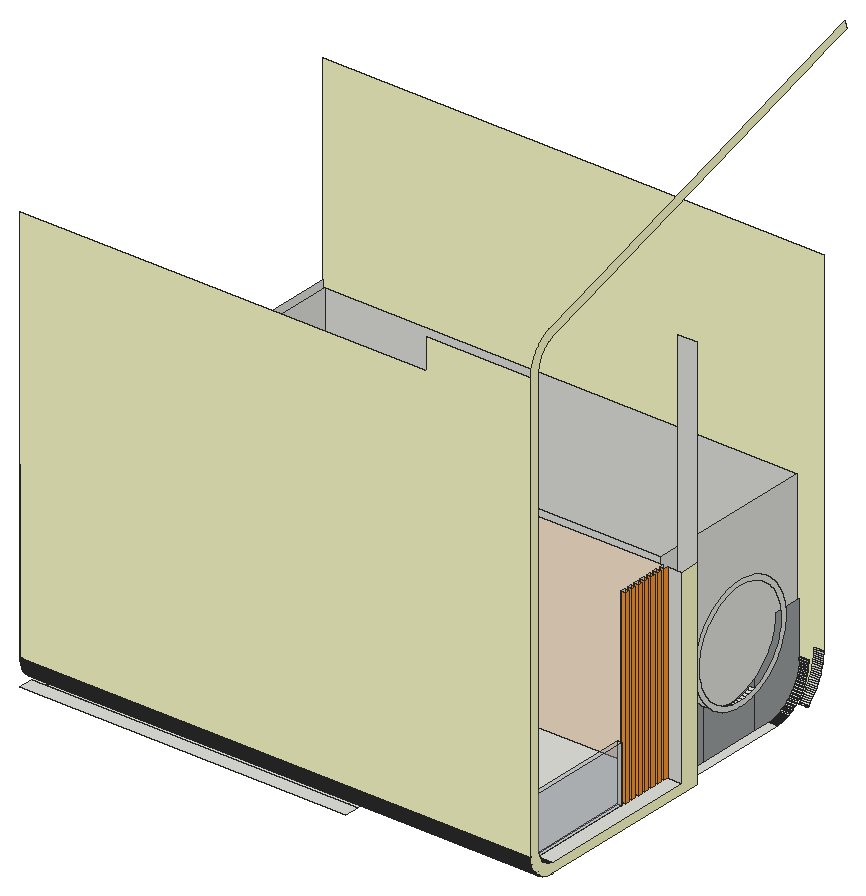
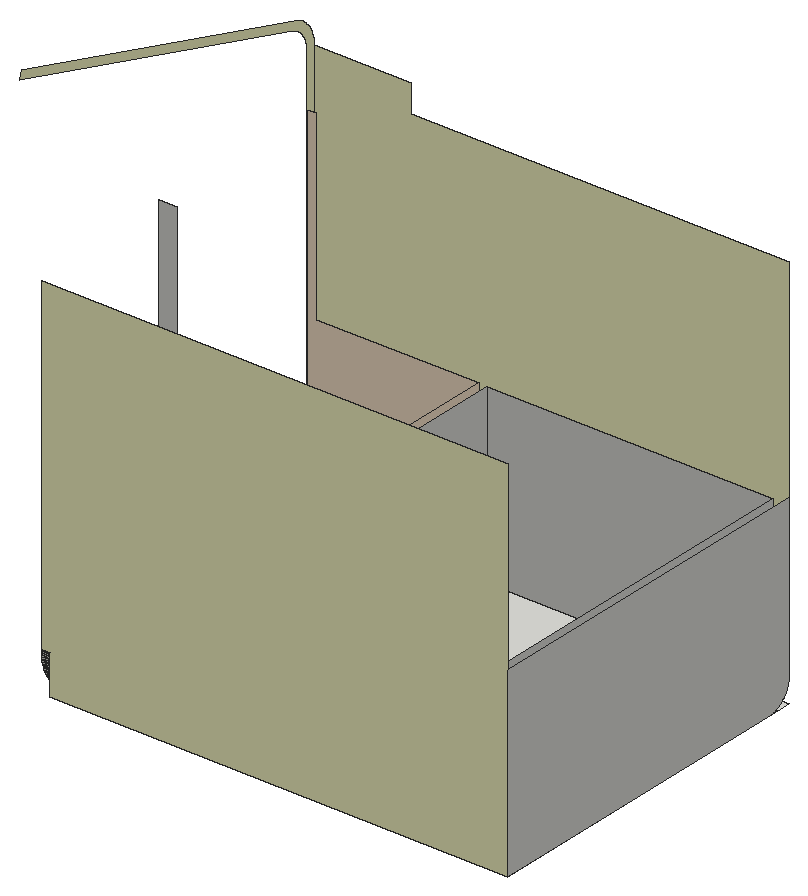
# SketchUp Ruby script. Lengths in inches.
U = 1.inch
M = Sketchup.active_model
def pt(a) = Geom::Point3d.new(a.map { |v| v * U })
def face(e, loops, mat)
  f = e.add_face(loops[0].map { |a| pt(a) })
  loops[1..].each { |l| e.add_face(l.map { |a| pt(a) }).erase! }
  f.material = f.back_material = mat if mat
  f
end
# faces: each face lists its corners as indices into pts; further lists are holes
def faces(e, pts, list, mat = nil) = list.each { |f| face(e, (f[0].is_a?(Array) ? f : [f]).map { |l| l.map { |i| pts[i] } }, mat) }
# xy, xz, yz: faces in a plane at the given z, y or x. An outline is a flat list of corners, or four numbers for a rectangle; further outlines are holes
def ring(l) = l.size == 4 ? [[l[0], l[1]], [l[2], l[1]], [l[2], l[3]], [l[0], l[3]]] : l.each_slice(2).to_a
def flat(e, list, mat, &to3) = list.each { |f| face(e, (f[0].is_a?(Array) ? f : [f]).map { |l| ring(l).map { |u, v| to3.(u, v) } }, mat) }
def xy(e, z, list, mat = nil) = flat(e, list, mat) { |x, y| [x, y, z] }
def xz(e, y, list, mat = nil) = flat(e, list, mat) { |x, z| [x, y, z] }
def yz(e, x, list, mat = nil) = flat(e, list, mat) { |y, z| [x, y, z] }
def lines(e, pts, list) = list.each { |a, b| e.add_line(pt(pts[a]), pt(pts[b])) }
# prism: a flat outline (further loops are holes) pulled along v
def prism(e, loops, v, mat = nil)
  f = face(e, loops, mat); d = Geom::Vector3d.new(v.map { |x| x * U })
  f.pushpull(f.normal.samedirection?(d) ? d.length : -d.length)
end
def box(e, o, s, mat = nil) = prism(e, [[o, [o[0] + s[0], o[1], o[2]], [o[0] + s[0], o[1] + s[1], o[2]], [o[0], o[1] + s[1], o[2]]]], [0, 0, s[2]], mat)
def at(x, y, z, deg = 0) = Geom::Transformation.translation(pt([x, y, z])) * Geom::Transformation.rotation(ORIGIN, Z_AXIS, deg.degrees)
def axes(o, x, y, z) = Geom::Transformation.new([*x, 0, *y, 0, *z, 0, *pt(o).to_a, 1])
def part(name) = M.definitions.add(name)
# library, detail: a bought-in or finely detailed component or shape, given as its bounding box
def library(name, o, s) = part(name).tap { |d| box(d.entities, o, s) }
def detail(e, o, s) = box(e.add_group.entities, o, s)
def put(e, d, t, mat = nil) = e.add_instance(d, t).tap { |i| i.material = mat if mat }
def group(e, t, mat = nil) = e.add_group.tap { |g| g.transformation = t; g.material = mat if mat }.entities
root = M.entities
M.materials.add("C03_Honey_Glow").color = [255, 234, 209]
M.materials.add("C04_Amber_Sunshine").color = [255, 152, 49]
M.materials.add("Denim_03_1K").color = [156, 160, 160]
M.materials.add("E01_Mint_Frost").color = [255, 255, 204]
M.materials.add("Glass_Basic_01").color = [161, 173, 186]
M.materials["Glass_Basic_01"].alpha = 0.25
c1 = library("porta+4",[0.2,-5.42,1.33],[46.55,4.72,83.21])
xy(root,126,[[5.5,15,212.5,24],[5.5,24,14.5,31.51],[14.5,24,206.5,31.51],[206.5,24,212.5,31.51],[5.5,31.51,14.5,255],
  [14.5,31.51,206.5,135],[206.5,31.51,212.5,135],[212.5,31.51,329.5,135],[14.5,135,206.5,141],[323.5,135,329.5,147],
  [14.5,141,206.5,246],[206.5,141,308.5,246],[317.5,147,323.5,219],[14.5,246,206.5,255]])
xy(root,132,[[11.5,21,206.5,21,206.5,141,311.5,141,311.5,249,11.5,249],[212.5,21,317.82,21,317.82,114.43,317.5,114.43,317.5,135,212.5,135],[320.5,33,329.5,33,329.5,135,320.5,135,320.5,132.43,317.5,132.43,317.5,129.86,320.5,129.86,320.5,127.29,317.5,127.29,317.5,124.71,320.5,124.71,320.5,122.14,317.5,122.14,317.5,119.57,320.5,119.57,320.5,117,317.5,117,317.5,114.43,320.5,114.43,320.5,111.86,317.82,111.86,317.82,109.29,320.5,109.29,320.5,106.71,317.82,106.71,317.82,104.14,320.5,104.14,320.5,101.57,317.82,101.57,317.82,99,320.5,99]])
xy(root,135,[[206.5,30,212.5,60]])
xz(root,15,[[5.5,142.51,329.5,142.51,329.5,415.29,263.5,415.29,263.5,396,5.5,396]],"E01_Mint_Frost")
xz(root,21,[[11.5,132,206.5,252]])
xz(root,21,[[212.5,132,212.5,252,323.5,252,323.5,378,329.5,378,329.5,144,320.5,144,320.5,168,317.82,168,317.82,132]],"C03_Honey_Glow")
xz(root,30,[[206.5,135,212.5,213]])
xz(root,60,[[206.5,135,212.5,213]])
xz(root,99,[[317.82,132,320.5,168]])
xz(root,101.57,[[317.82,132,320.5,252]],"C04_Amber_Sunshine")
xz(root,104.14,[[317.82,132,320.5,252]],"C04_Amber_Sunshine")
xz(root,106.71,[[317.82,132,320.5,252]],"C04_Amber_Sunshine")
xz(root,109.29,[[317.82,132,320.5,252]],"C04_Amber_Sunshine")
xz(root,111.86,[[317.82,132,320.5,252]],"C04_Amber_Sunshine")
xz(root,114.43,[[317.82,132,320.5,252]],"C04_Amber_Sunshine")
xz(root,117,[[317.5,132,320.5,252]],"C04_Amber_Sunshine")
xz(root,119.57,[[317.5,132,320.5,252]],"C04_Amber_Sunshine")
xz(root,122.14,[[317.5,132,320.5,252]],"C04_Amber_Sunshine")
xz(root,124.71,[[317.5,132,320.5,252]],"C04_Amber_Sunshine")
xz(root,127.29,[[317.5,132,320.5,252]],"C04_Amber_Sunshine")
xz(root,129.86,[[317.5,132,320.5,252]],"C04_Amber_Sunshine")
xz(root,132.43,[[317.5,132,320.5,252]],"C04_Amber_Sunshine")
xz(root,135,[[320.5,132,329.5,252]])
xz(root,135,[[212.5,132,317.5,252]],"C03_Honey_Glow")
xz(root,141,[[206.5,132,311.5,252]])
xz(root,147,[[317.5,126,329.5,378]])
xz(root,243,[[317.5,150.6,323.5,150.75]])
xz(root,243.02,[[317.5,151.4,323.5,152.2]])
xz(root,249,[[11.5,132,311.5,252]])
xz(root,255,[[5.5,126,5.5,378,323.5,378,323.5,153,317.5,153,317.5,126]],"E01_Mint_Frost")
yz(root,5.5,[[31.51,126,31.28,126.01,30.71,126.05,30.14,126.11,29.57,126.1875,29.01,126.29,28.45,126.4,27.89,126.54,27.34,126.69,26.8,126.86,26.25,127.05,25.72,127.26,25.19,127.48,24.68,127.72,24.16,127.98,23.66,128.26,23.17,128.55,22.6875,128.86,22.22,129.1875,21.76,129.53,21.31,129.88,20.87,130.25,20.03,131.03,19.25,131.87,18.88,132.31,18.53,132.76,18.1875,133.22,17.86,133.6875,17.55,134.17,17.26,134.66,16.98,135.16,16.72,135.68,16.48,136.19,16.26,136.72,16.05,137.25,15.86,137.8,15.69,138.34,15.54,138.89,15.4,139.45,15.29,140.01,15.1875,140.57,15.11,141.14,15.05,141.71,15.01,142.28,15,142.51,15,252,255,252,255,126]])
yz(root,11.5,[[21,132,249,252]])
yz(root,206.5,[[[21,132,141,252],[30,135,60,213],[78,171,120,213]]])
yz(root,212.5,[[[27,132,63,216],[30,135,60,213]]])
yz(root,212.5,[[[21,132,27,132,27,216,63,216,63,132,135,132,135,252,21,252],[75,168,123,216]]],"C03_Honey_Glow")
yz(root,311.5,[[141,132,249,252]])
yz(root,317.5,[[242.99,126,243,126,243,126.01],[117,132,119.57,252],[122.14,132,124.71,252],[127.29,132,129.86,252],[132.43,132,135,252],
  [243,150.75,243.02,151.4,243.02,152.2,243,153]])
yz(root,317.5,[[147,126,167.18,126,167.18,157.37,165.42,158.8,163.76,160.33,162.2,161.97,160.74,163.7,159.4,165.51,158.17,167.41,157.0625,169.39,156.08,171.42,155.23,173.52,154.52,175.67,153.93,177.85,153.49,180.07,153.19,182.31,153.03,184.57,147,184.57],[167.18,126,207.59,126,207.59,155.17,205.61,154.0625,203.58,153.08,201.48,152.23,199.33,151.52,197.15,150.93,194.93,150.49,192.69,150.19,190.43,150.03,188.17,150.01,185.91,150.13,183.67,150.4,181.44,150.8,179.25,151.35,177.09,152.03,174.98,152.84,172.93,153.79,170.9375,154.86,169.02,156.06,167.18,157.37],[207.59,126,219,126,219.8,126.07,220.59,126.17,221.38,126.29,222.17,126.43,222.95,126.6,223.72,126.79,224.49,127.01,225.26,127.25,226.01,127.51,226.76,127.8,227.49,128.1,228.22,128.4375,228.9375,128.79,229.64,129.17,230.34,129.5625,231.02,129.98,231.6875,130.42,232.34,130.88,232.98,131.36,233.6,131.86,234.21,132.38,234.8,132.91,235.38,133.47,235.9375,134.04,236.48,134.63,237,135.24,237.5,135.86,237.99,136.49,238.45,137.15,238.89,137.8125,239.32,138.49,239.72,139.18,240.1,139.88,240.45,140.6,240.79,141.32,241.1,142.06,241.39,142.8,241.66,143.56,241.91,144.32,242.125,145.09,242.32,145.86,242.5,146.64,242.64,147.43,242.77,148.22,242.87,149.01,242.94,149.81,243,150.6,243,185.17,224.99,185.17,224.87,182.91,224.6,180.67,224.2,178.44,223.65,176.25,222.97,174.09,222.16,171.98,221.21,169.93,220.14,167.9375,218.94,166.02,217.63,164.18,216.2,162.42,214.67,160.76,213.03,159.2,211.3,157.74,209.49,156.4,207.59,155.17]],"Denim_03_1K")
yz(root,317.82,[[101.57,132,104.14,252],[106.71,132,109.29,252],[111.86,132,114.43,252]])
yz(root,317.82,[[21,132,99,168]],"Glass_Basic_01")
yz(root,320.5,[[101.57,132,104.14,252],[106.71,132,109.29,252],[111.86,132,114.43,252],[117,132,119.57,252],[122.14,132,124.71,252],
  [127.29,132,129.86,252],[132.43,132,135,252]],"C04_Amber_Sunshine")
yz(root,320.5,[[33,132,99,132,99,168,21,168,21,144,21.04,143.63,21.09,143.27,21.15,142.91,21.22,142.55,21.3,142.1875,21.39,141.83,21.49,141.48,21.6,141.125,21.72,140.78,21.85,140.43,22.13,139.75,22.29,139.42,22.46,139.09,22.63,138.77,22.8125,138.45,23.01,138.14,23.21,137.83,23.42,137.53,23.64,137.23,23.86,136.9375,24.1,136.65,24.34,136.375,24.59,136.11,24.84,135.84,25.11,135.59,25.375,135.34,25.65,135.1,25.9375,134.86,26.23,134.64,26.53,134.42,26.83,134.21,27.14,134.01,27.45,133.8125,27.77,133.63,28.09,133.46,28.42,133.29,28.75,133.13,29.43,132.85,29.78,132.72,30.125,132.6,30.48,132.49,30.83,132.39,31.1875,132.3,31.55,132.22,31.91,132.15,32.27,132.09,32.63,132.04]],"Glass_Basic_01")
yz(root,323.5,[[[188.17,150.01,190.43,150.03,192.69,150.19,194.93,150.49,197.15,150.93,199.33,151.52,201.48,152.23,203.58,153.08,205.61,154.0625,207.59,155.17,209.49,156.4,211.3,157.74,213.03,159.2,214.67,160.76,216.2,162.42,217.63,164.18,218.94,166.02,220.14,167.9375,221.21,169.93,222.16,171.98,222.97,174.09,223.65,176.25,224.2,178.44,224.6,180.67,224.87,182.91,224.99,185.17,224.97,187.43,224.81,189.69,224.51,191.93,224.07,194.15,223.48,196.33,222.77,198.48,221.92,200.58,220.9375,202.61,219.83,204.59,218.6,206.49,217.26,208.3,215.8,210.03,214.24,211.67,212.58,213.2,210.82,214.63,208.98,215.94,207.0625,217.14,205.07,218.21,203.02,219.16,200.91,219.97,198.75,220.65,196.56,221.2,194.33,221.6,192.09,221.87,189.83,221.99,187.57,221.97,185.31,221.81,183.07,221.51,180.85,221.07,178.67,220.48,176.52,219.77,174.42,218.92,172.39,217.9375,170.41,216.83,168.51,215.6,166.7,214.26,164.97,212.8,163.33,211.24,161.8,209.58,160.37,207.82,159.06,205.98,157.86,204.0625,156.79,202.07,155.84,200.02,155.03,197.91,154.35,195.75,153.8,193.56,153.4,191.33,153.13,189.09,153.01,186.83,153.03,184.57,153.19,182.31,153.49,180.07,153.93,177.85,154.52,175.67,155.23,173.52,156.08,171.42,157.0625,169.39,158.17,167.41,159.4,165.51,160.74,163.7,162.2,161.97,163.76,160.33,165.42,158.8,167.18,157.37,169.02,156.06,170.9375,154.86,172.93,153.79,174.98,152.84,177.09,152.03,179.25,151.35,181.44,150.8,183.67,150.4,185.91,150.13],[188.24,153.01,186.17,153.12,184.11,153.36,182.07,153.74,180.0625,154.23,178.08,154.86,176.15,155.6,174.27,156.47,172.44,157.45,170.68,158.55,168.99,159.76,167.39,161.0625,165.86,162.47,164.43,163.97,163.1,165.55,161.86,167.22,160.74,168.96,159.72,170.77,158.83,172.64,158.05,174.56,157.39,176.53,156.86,178.53,156.45,180.5625,156.17,182.62,156.03,184.69,156.01,186.76,156.12,188.83,156.36,190.89,156.74,192.93,157.23,194.9375,157.86,196.92,158.6,198.85,159.47,200.73,160.45,202.56,161.55,204.32,162.76,206.01,164.0625,207.61,165.47,209.14,166.97,210.57,168.55,211.9,170.22,213.14,171.96,214.26,173.77,215.28,175.64,216.17,177.56,216.95,179.53,217.61,181.53,218.14,183.5625,218.55,185.62,218.83,187.69,218.97,189.76,218.99,191.83,218.88,193.89,218.64,195.93,218.26,197.9375,217.77,199.92,217.14,201.85,216.4,203.73,215.53,205.56,214.55,207.32,213.45,209.01,212.24,210.61,210.9375,212.14,209.53,213.57,208.03,214.9,206.45,216.14,204.78,217.26,203.04,218.28,201.23,219.17,199.36,219.95,197.44,220.61,195.47,221.14,193.47,221.55,191.4375,221.83,189.38,221.97,187.31,221.99,185.24,221.88,183.17,221.64,181.11,221.26,179.07,220.77,177.0625,220.14,175.08,219.4,173.15,218.53,171.27,217.55,169.44,216.45,167.68,215.24,165.99,213.9375,164.39,212.53,162.86,211.03,161.43,209.45,160.1,207.78,158.86,206.04,157.74,204.23,156.72,202.36,155.83,200.44,155.05,198.47,154.39,196.47,153.86,194.4375,153.45,192.38,153.17,190.31,153.03]]])
yz(root,329.5,[[32.43,125.98,33,126,31.51,126,31.85,125.99],[15,142.51,15,144,14.98,143.43,14.99,142.85]])
yz(root,329.5,[[31.51,126,147,126,147,252,135,252,135,132,33,132,32.63,132.04,32.27,132.09,31.91,132.15,31.55,132.22,31.1875,132.3,30.83,132.39,30.48,132.49,30.125,132.6,29.78,132.72,29.43,132.85,28.75,133.13,28.42,133.29,28.09,133.46,27.77,133.63,27.45,133.8125,27.14,134.01,26.83,134.21,26.53,134.42,26.23,134.64,25.9375,134.86,25.65,135.1,25.375,135.34,25.11,135.59,24.84,135.84,24.59,136.11,24.34,136.375,24.1,136.65,23.86,136.9375,23.64,137.23,23.42,137.53,23.21,137.83,23.01,138.14,22.8125,138.45,22.63,138.77,22.46,139.09,22.29,139.42,22.13,139.75,21.85,140.43,21.72,140.78,21.6,141.125,21.49,141.48,21.39,141.83,21.3,142.1875,21.22,142.55,21.15,142.91,21.09,143.27,21.04,143.63,21,144,21,414,20.99,414.47,20.99,414.95,21,415.2,21.01,415.42,21.03,415.9,21.07,416.37,21.125,416.84,21.19,417.31,21.27,417.78,21.36,418.24,21.46,418.71,21.57,419.17,21.7,419.625,21.84,420.08,21.99,420.53,22.15,420.97,22.32,421.41,22.51,421.85,22.7,422.28,22.91,422.71,23.13,423.13,23.36,423.54,23.6,423.95,23.85,424.35,24.11,424.75,24.39,425.14,24.67,425.52,24.96,425.89,25.26,426.26,25.9,426.96,26.23,427.3,26.57,427.64,26.91,427.96,27.63,428.58,28.01,428.87,28.77,429.43,29.17,429.69,29.57,429.94,29.98,430.1875,30.39,430.42,30.81,430.64,31.23,430.85,31.67,431.05,32.1,431.23,32.54,431.41,32.99,431.57,33.4375,431.72,57,439.04,247,498,247,498.15,265.85,504,264.19,509.34,30.96,436.95,30.41,436.76,29.83,436.54,29.25,436.3,28.68,436.04,28.12,435.77,27.56,435.49,27.01,435.19,26.47,434.88,25.9375,434.55,25.42,434.21,24.9,433.85,24.4,433.49,23.9,433.1,23.42,432.71,22.95,432.3,22.49,431.88,22.03,431.45,21.59,431.01,20.75,430.09,20.35,429.61,19.96,429.12,19.58,428.625,19.22,428.12,18.87,427.6,18.53,427.07,18.21,426.54,17.9,426,17.61,425.44,17.33,424.89,17.07,424.32,16.82,423.75,16.58,423.17,16.16,421.99,15.98,421.4,15.81,420.8,15.65,420.19,15.51,419.58,15.39,418.97,15.28,418.36,15.19,417.74,15.12,417.12,15.0625,416.5,15.02,415.87,15,415.29,15,142.51,15.01,142.28,15.05,141.71,15.11,141.14,15.1875,140.57,15.29,140.01,15.4,139.45,15.54,138.89,15.69,138.34,15.86,137.8,16.05,137.25,16.26,136.72,16.48,136.19,16.72,135.68,16.98,135.16,17.26,134.66,17.55,134.17,17.86,133.6875,18.1875,133.22,18.53,132.76,18.88,132.31,19.25,131.87,20.03,131.03,20.87,130.25,21.31,129.88,21.76,129.53,22.22,129.1875,22.6875,128.86,23.17,128.55,23.66,128.26,24.16,127.98,24.68,127.72,25.19,127.48,25.72,127.26,26.25,127.05,26.8,126.86,27.34,126.69,27.89,126.54,28.45,126.4,29.01,126.29,29.57,126.1875,30.14,126.11,30.71,126.05,31.28,126.01]],"E01_Mint_Frost")
p = [[317.5,242.89,125.91],[317.5,242.99,126],[323.5,242.99,126],[323.5,242.89,125.91],[329.5,30.71,126.05],[329.5,30.14,126.11],
  [5.5,30.14,126.11],[5.5,30.71,126.05],[329.5,31.28,126.01],[5.5,31.28,126.01],[329.5,31.51,126],[5.5,31.51,126],
  [14.5,31.51,126],[206.5,31.51,126],[212.5,31.51,126],[317.5,219.8,126.07],[317.5,219,126],[323.5,219,126],
  [323.5,219.8,126.07],[317.5,243,126.01],[323.5,243,126.01],[317.5,243.73,126.67],[323.5,243.73,126.67],[329.5,29.57,126.1875],
  [5.5,29.57,126.1875],[317.5,220.59,126.17],[323.5,220.59,126.17],[329.5,29.01,126.29],[5.5,29.01,126.29],[317.5,221.38,126.29],
  [323.5,221.38,126.29],[329.5,28.45,126.4],[5.5,28.45,126.4],[317.5,222.17,126.43],[323.5,222.17,126.43],[329.5,27.89,126.54],
  [5.5,27.89,126.54],[317.5,222.95,126.6],[323.5,222.95,126.6],[329.5,27.34,126.69],[5.5,27.34,126.69],[317.5,223.72,126.79],
  [323.5,223.72,126.79],[329.5,26.8,126.86],[5.5,26.8,126.86],[317.5,244.54,127.46],[323.5,244.54,127.46],[317.5,224.49,127.01],
  [323.5,224.49,127.01],[329.5,26.25,127.05],[5.5,26.25,127.05],[317.5,225.26,127.25],[323.5,225.26,127.25],[329.5,25.72,127.26],
  [5.5,25.72,127.26],[317.5,226.01,127.51],[323.5,226.01,127.51],[329.5,25.19,127.48],[5.5,25.19,127.48],[329.5,24.68,127.72],
  [5.5,24.68,127.72],[317.5,226.76,127.8],[323.5,226.76,127.8],[317.5,245.33,128.27],[323.5,245.33,128.27],[329.5,24.16,127.98],
  [5.5,24.16,127.98],[317.5,227.49,128.1],[323.5,227.49,128.1],[329.5,23.66,128.26],[5.5,23.66,128.26],[317.5,228.22,128.4375],
  [323.5,228.22,128.4375],[329.5,23.17,128.55],[5.5,23.17,128.55],[317.5,246.09,129.11],[323.5,246.09,129.11],[317.5,228.9375,128.79],
  [323.5,228.9375,128.79],[329.5,22.6875,128.86],[5.5,22.6875,128.86],[317.5,229.64,129.17],[323.5,229.64,129.17],[329.5,22.22,129.1875],
  [5.5,22.22,129.1875],[317.5,246.83,129.98],[323.5,246.83,129.98],[329.5,21.76,129.53],[5.5,21.76,129.53],[317.5,230.34,129.5625],
  [323.5,230.34,129.5625],[329.5,21.31,129.88],[5.5,21.31,129.88],[317.5,231.02,129.98],[323.5,231.02,129.98],[329.5,20.87,130.25],
  [5.5,20.87,130.25],[317.5,231.6875,130.42],[323.5,231.6875,130.42],[317.5,247.53,130.86],[323.5,247.53,130.86],[329.5,20.45,130.64],
  [5.5,20.45,130.64],[317.5,232.34,130.88],[323.5,232.34,130.88],[329.5,20.03,131.03],[5.5,20.03,131.03],[317.5,232.98,131.36],
  [323.5,232.98,131.36],[317.5,248.21,131.77],[323.5,248.21,131.77],[329.5,19.64,131.45],[5.5,19.64,131.45],[329.5,19.25,131.87],
  [5.5,19.25,131.87],[317.5,233.6,131.86],[323.5,233.6,131.86],[317.5,248.86,132.7],[323.5,248.86,132.7],[329.5,18.88,132.31],
  [5.5,18.88,132.31],[317.5,234.21,132.38],[323.5,234.21,132.38],[329.5,32.27,132.09],[329.5,32.63,132.04],[320.5,32.63,132.04],
  [320.5,32.27,132.09],[329.5,33,132],[320.5,33,132],[329.5,31.91,132.15],[320.5,31.91,132.15],[329.5,31.1875,132.3],
  [329.5,31.55,132.22],[320.5,31.55,132.22],[320.5,31.1875,132.3],[329.5,18.53,132.76],[5.5,18.53,132.76],[329.5,30.83,132.39],
  [320.5,30.83,132.39],[329.5,30.48,132.49],[320.5,30.48,132.49],[317.5,234.8,132.91],[323.5,234.8,132.91],[329.5,30.125,132.6],
  [320.5,30.125,132.6],[329.5,29.78,132.72],[320.5,29.78,132.72],[329.5,29.43,132.85],[320.5,29.43,132.85],[317.5,249.48,133.65],
  [323.5,249.48,133.65],[329.5,18.1875,133.22],[5.5,18.1875,133.22],[329.5,29.09,132.99],[320.5,29.09,132.99],[317.5,235.38,133.47],
  [323.5,235.38,133.47],[329.5,28.75,133.13],[320.5,28.75,133.13],[329.5,28.42,133.29],[320.5,28.42,133.29],[329.5,17.86,133.6875],
  [5.5,17.86,133.6875],[329.5,28.09,133.46],[320.5,28.09,133.46],[329.5,27.77,133.63],[320.5,27.77,133.63],[317.5,235.9375,134.04],
  [323.5,235.9375,134.04],[329.5,27.45,133.8125],[320.5,27.45,133.8125],[317.5,250.07,134.61],[323.5,250.07,134.61],[329.5,17.55,134.17],
  [5.5,17.55,134.17],[329.5,27.14,134.01],[320.5,27.14,134.01],[329.5,26.83,134.21],[320.5,26.83,134.21],[317.5,236.48,134.63],
  [323.5,236.48,134.63],[329.5,17.26,134.66],[5.5,17.26,134.66],[329.5,26.53,134.42],[320.5,26.53,134.42],[329.5,26.23,134.64],
  [320.5,26.23,134.64],[329.5,25.9375,134.86],[320.5,25.9375,134.86],[317.5,237,135.24],[323.5,237,135.24],[317.5,250.63,135.6],
  [323.5,250.63,135.6],[329.5,16.98,135.16],[5.5,16.98,135.16],[329.5,25.65,135.1],[320.5,25.65,135.1],[329.5,25.375,135.34],
  [320.5,25.375,135.34],[329.5,16.72,135.68],[5.5,16.72,135.68],[317.5,237.5,135.86],[323.5,237.5,135.86],[329.5,25.11,135.59],
  [320.5,25.11,135.59],[329.5,24.84,135.84],[320.5,24.84,135.84],[317.5,251.16,136.6],[323.5,251.16,136.6],[329.5,16.48,136.19],
  [5.5,16.48,136.19],[329.5,24.59,136.11],[320.5,24.59,136.11],[317.5,237.99,136.49],[323.5,237.99,136.49],[329.5,24.34,136.375],
  [320.5,24.34,136.375],[329.5,16.26,136.72],[5.5,16.26,136.72],[329.5,24.1,136.65],[320.5,24.1,136.65],[317.5,238.45,137.15],
  [323.5,238.45,137.15],[317.5,251.65,137.62],[323.5,251.65,137.62],[329.5,16.05,137.25],[5.5,16.05,137.25],[329.5,23.86,136.9375],
  [320.5,23.86,136.9375],[329.5,23.64,137.23],[320.5,23.64,137.23],[317.5,238.89,137.8125],[323.5,238.89,137.8125],[329.5,23.42,137.53],
  [320.5,23.42,137.53],[329.5,15.86,137.8],[5.5,15.86,137.8],[329.5,23.21,137.83],[320.5,23.21,137.83],[317.5,252.12,138.66],
  [323.5,252.12,138.66],[329.5,15.69,138.34],[5.5,15.69,138.34],[329.5,23.01,138.14],[320.5,23.01,138.14],[317.5,239.32,138.49],
  [323.5,239.32,138.49],[329.5,22.8125,138.45],[320.5,22.8125,138.45],[329.5,15.54,138.89],[5.5,15.54,138.89],[329.5,22.63,138.77],
  [320.5,22.63,138.77],[317.5,239.72,139.18],[323.5,239.72,139.18],[317.5,252.55,139.71],[323.5,252.55,139.71],[329.5,22.46,139.09],
  [320.5,22.46,139.09],[329.5,15.4,139.45],[5.5,15.4,139.45],[329.5,22.29,139.42],[320.5,22.29,139.42],[317.5,240.1,139.88],
  [323.5,240.1,139.88],[329.5,15.29,140.01],[5.5,15.29,140.01],[329.5,22.13,139.75],[320.5,22.13,139.75],[317.5,252.94,140.77],
  [323.5,252.94,140.77],[329.5,21.99,140.09],[320.5,21.99,140.09],[317.5,240.45,140.6],[323.5,240.45,140.6],[329.5,15.1875,140.57],
  [5.5,15.1875,140.57],[329.5,21.85,140.43],[320.5,21.85,140.43],[329.5,21.72,140.78],[320.5,21.72,140.78],[329.5,15.11,141.14],
  [5.5,15.11,141.14],[317.5,240.79,141.32],[323.5,240.79,141.32],[329.5,21.6,141.125],[320.5,21.6,141.125],[317.5,253.3,141.84],
  [323.5,253.3,141.84],[329.5,15.05,141.71],[5.5,15.05,141.71],[329.5,21.49,141.48],[320.5,21.49,141.48],[317.5,241.1,142.06],
  [323.5,241.1,142.06],[329.5,21.39,141.83],[320.5,21.39,141.83],[329.5,15.01,142.28],[5.5,15.01,142.28],[329.5,21.3,142.1875],
  [320.5,21.3,142.1875],[317.5,253.63,142.93],[323.5,253.63,142.93],[317.5,241.39,142.8],[323.5,241.39,142.8],[329.5,21.22,142.55],
  [320.5,21.22,142.55],[329.5,15,142.51],[5.5,15,142.51],[329.5,21.15,142.91],[320.5,21.15,142.91],[317.5,241.66,143.56],
  [323.5,241.66,143.56],[329.5,21.09,143.27],[320.5,21.09,143.27],[317.5,253.93,144.02],[323.5,253.93,144.02],[329.5,21.04,143.63],
  [320.5,21.04,143.63],[329.5,21,144],[320.5,21,144],[317.5,241.91,144.32],[323.5,241.91,144.32],[317.5,254.18,145.125],
  [323.5,254.18,145.125],[317.5,242.125,145.09],[323.5,242.125,145.09],[317.5,242.32,145.86],[323.5,242.32,145.86],[317.5,254.41,146.24],
  [323.5,254.41,146.24],[317.5,242.5,146.64],[323.5,242.5,146.64],[317.5,254.6,147.35],[323.5,254.6,147.35],[317.5,242.64,147.43],
  [323.5,242.64,147.43],[317.5,242.77,148.22],[323.5,242.77,148.22],[317.5,254.75,148.48],[323.5,254.75,148.48],[317.5,242.87,149.01],
  [323.5,242.87,149.01],[317.5,254.87,149.6],[323.5,254.87,149.6],[317.5,242.94,149.81],[323.5,242.94,149.81],[317.5,254.95,150.73],
  [323.5,254.95,150.73],[317.5,243,150.6],[323.5,243,150.6],[317.5,185.91,150.13],[317.5,188.17,150.01],[323.5,188.17,150.01],
  [323.5,185.91,150.13],[317.5,190.43,150.03],[323.5,190.43,150.03],[317.5,192.69,150.19],[323.5,192.69,150.19],[317.5,183.67,150.4],
  [323.5,183.67,150.4],[317.5,194.93,150.49],[323.5,194.93,150.49],[317.5,181.44,150.8],[323.5,181.44,150.8],[317.5,197.15,150.93],
  [323.5,197.15,150.93],[317.5,243.02,151.4],[317.5,243,150.75],[323.5,243,150.75],[323.5,243.02,151.4],[317.5,254.99,151.87],
  [323.5,254.99,151.87],[317.5,179.25,151.35],[323.5,179.25,151.35],[317.5,199.33,151.52],[323.5,199.33,151.52],[317.5,177.09,152.03],
  [323.5,177.09,152.03],[317.5,201.48,152.23],[323.5,201.48,152.23],[317.5,255,153],[323.5,255,153],[317.5,174.98,152.84],
  [323.5,174.98,152.84],[317.5,203.58,153.08],[323.5,203.58,153.08],[317.5,243,153],[317.5,243.02,152.2],[323.5,243.02,152.2],
  [323.5,243,153],[308.5,246,126],[317.5,246,126],[212.5,135,126],[212.5,135,132],[329.5,21,132],
  [320.5,21,132]]
faces(root,p,[[0,1,2,3],[15,16,17,18],[1,19,20,2],[19,21,22,20],[25,15,18,26],[29,25,26,30],[33,29,30,34],[37,33,34,38],
  [41,37,38,42],[21,45,46,22],[47,41,42,48],[51,47,48,52],[55,51,52,56],[61,55,56,62],[45,63,64,46],[67,61,62,68],
  [71,67,68,72],[63,75,76,64],[77,71,72,78],[81,77,78,82],[75,85,86,76],[89,81,82,90],[93,89,90,94],[97,93,94,98],
  [85,99,100,86],[103,97,98,104],[107,103,104,108],[99,109,110,100],[115,107,108,116],[109,117,118,110],[121,115,116,122],[123,124,125,126],
  [124,127,128,125],[129,123,126,130],[131,132,133,134],[132,129,130,133],[137,131,134,138],[139,137,138,140],[141,121,122,142],[143,139,140,144],
  [145,143,144,146],[147,145,146,148],[117,149,150,118],[153,147,148,154],[155,141,142,156],[157,153,154,158],[159,157,158,160],[163,159,160,164],
  [165,163,164,166],[167,155,156,168],[169,165,166,170],[149,171,172,150],[175,169,170,176],[177,175,176,178],[179,167,168,180],[183,177,178,184],
  [185,183,184,186],[187,185,186,188],[189,179,180,190],[171,191,192,172],[195,187,188,196],[197,195,196,198],[201,189,190,202],[203,197,198,204],
  [205,203,204,206],[191,207,208,192],[211,205,206,212],[213,201,202,214],[215,211,212,216],[219,215,216,220],[221,213,214,222],[207,223,224,208],
  [227,219,220,228],[229,227,228,230],[231,221,222,232],[233,229,230,234],[237,233,234,238],[223,239,240,224],[243,237,238,244],[245,231,232,246],
  [247,243,244,248],[251,247,248,252],[253,245,246,254],[239,255,256,240],[257,251,252,258],[261,257,258,262],[263,253,254,264],[267,261,262,268],
  [255,269,270,256],[271,267,268,272],[273,263,264,274],[277,271,272,278],[279,277,278,280],[283,273,274,284],[285,279,280,286],[269,287,288,270],
  [291,285,286,292],[293,283,284,294],[295,291,292,296],[299,295,296,300],[287,301,302,288],[303,293,294,304],[305,299,300,306],[309,305,306,310],
  [311,303,304,312],[313,309,310,314],[301,315,316,302],[317,313,314,318],[319,317,318,320],[321,311,312,322],[315,323,324,316],[325,321,322,326],
  [327,325,326,328],[323,329,330,324],[331,327,328,332],[329,333,334,330],[335,331,332,336],[337,335,336,338],[333,339,340,334],[341,337,338,342],
  [339,343,344,340],[345,341,342,346],[343,347,348,344],[349,345,346,350],[351,352,353,354],[352,355,356,353],[355,357,358,356],[359,351,354,360],
  [357,361,362,358],[363,359,360,364],[361,365,366,362],[367,368,369,370],[347,371,372,348],[373,363,364,374],[365,375,376,366],[377,373,374,378],
  [375,379,380,376],[371,381,382,372],[383,377,378,384],[379,385,386,380],[387,388,389,390]])
faces(root,p,[[4,5,6,7],[8,4,7,9],[10,8,9,11,12,13,14],[5,23,24,6],[23,27,28,24],[27,31,32,28],[31,35,36,32],[35,39,40,36],
  [39,43,44,40],[43,49,50,44],[49,53,54,50],[53,57,58,54],[57,59,60,58],[59,65,66,60],[65,69,70,66],[69,73,74,70],
  [73,79,80,74],[79,83,84,80],[83,87,88,84],[87,91,92,88],[91,95,96,92],[95,101,102,96],[101,105,106,102],[105,111,112,106],
  [111,113,114,112],[113,119,120,114],[119,135,136,120],[135,151,152,136],[151,161,162,152],[161,173,174,162],[173,181,182,174],[181,193,194,182],
  [193,199,200,194],[199,209,210,200],[209,217,218,210],[217,225,226,218],[225,235,236,226],[235,241,242,236],[241,249,250,242],[249,259,260,250],
  [259,265,266,260],[265,275,276,266],[275,281,282,276],[281,289,290,282],[289,297,298,290],[297,307,308,298]],"E01_Mint_Frost")
lines(root,p,[[391,392],[393,394],[395,396],[320,396],[128,396]])
put(root,c1,axes([209.72,26.84,130.64],[0,0.77339,0],[-1,0,0],[0,0,1]))
